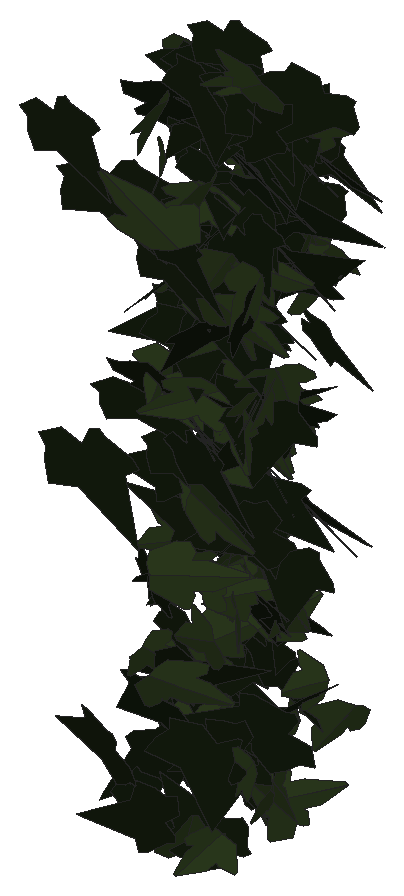
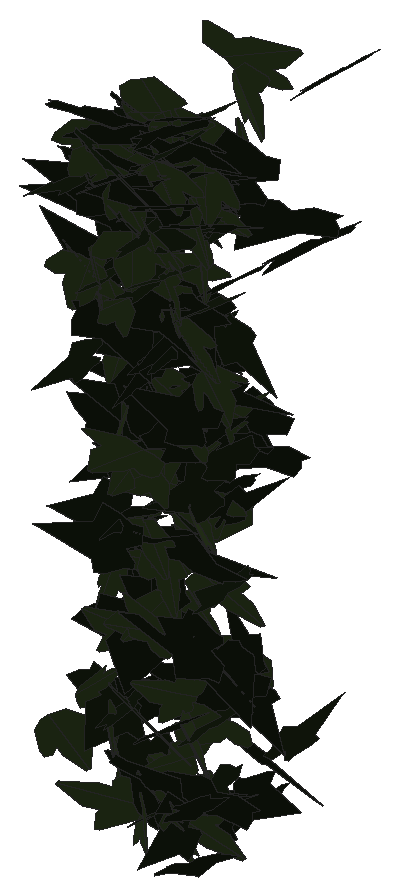
# SketchUp Ruby script. Lengths in millimetres.
U = 1.mm
M = Sketchup.active_model
def pt(a) = Geom::Point3d.new(a.map { |v| v * U })
def face(e, loops, mat)
  f = e.add_face(loops[0].map { |a| pt(a) })
  loops[1..].each { |l| e.add_face(l.map { |a| pt(a) }).erase! }
  f.material = f.back_material = mat if mat
  f
end
# faces: each face lists its corners as indices into pts; further lists are holes
def faces(e, pts, list, mat = nil) = list.each { |f| face(e, (f[0].is_a?(Array) ? f : [f]).map { |l| l.map { |i| pts[i] } }, mat) }
# xy, xz, yz: faces in a plane at the given z, y or x. An outline is a flat list of corners, or four numbers for a rectangle; further outlines are holes
def ring(l) = l.size == 4 ? [[l[0], l[1]], [l[2], l[1]], [l[2], l[3]], [l[0], l[3]]] : l.each_slice(2).to_a
def flat(e, list, mat, &to3) = list.each { |f| face(e, (f[0].is_a?(Array) ? f : [f]).map { |l| ring(l).map { |u, v| to3.(u, v) } }, mat) }
def xy(e, z, list, mat = nil) = flat(e, list, mat) { |x, y| [x, y, z] }
def xz(e, y, list, mat = nil) = flat(e, list, mat) { |x, z| [x, y, z] }
def yz(e, x, list, mat = nil) = flat(e, list, mat) { |y, z| [x, y, z] }
def lines(e, pts, list) = list.each { |a, b| e.add_line(pt(pts[a]), pt(pts[b])) }
# prism: a flat outline (further loops are holes) pulled along v
def prism(e, loops, v, mat = nil)
  f = face(e, loops, mat); d = Geom::Vector3d.new(v.map { |x| x * U })
  f.pushpull(f.normal.samedirection?(d) ? d.length : -d.length)
end
def box(e, o, s, mat = nil) = prism(e, [[o, [o[0] + s[0], o[1], o[2]], [o[0] + s[0], o[1] + s[1], o[2]], [o[0], o[1] + s[1], o[2]]]], [0, 0, s[2]], mat)
def at(x, y, z, deg = 0) = Geom::Transformation.translation(pt([x, y, z])) * Geom::Transformation.rotation(ORIGIN, Z_AXIS, deg.degrees)
def axes(o, x, y, z) = Geom::Transformation.new([*x, 0, *y, 0, *z, 0, *pt(o).to_a, 1])
def part(name) = M.definitions.add(name)
# library, detail: a bought-in or finely detailed component or shape, given as its bounding box
def library(name, o, s) = part(name).tap { |d| box(d.entities, o, s) }
def detail(e, o, s) = box(e.add_group.entities, o, s)
def put(e, d, t, mat = nil) = e.add_instance(d, t).tap { |i| i.material = mat if mat }
def group(e, t, mat = nil) = e.add_group.tap { |g| g.transformation = t; g.material = mat if mat }.entities
root = M.entities
M.materials.add("efeu1").color = [18, 25, 13]
M.materials.add("efeu2").color = [43, 57, 29]
c1 = part("ivyleaf_9")
p = [[39.1,54.8,31.7],[34.5,51.8,30.2],[-5.3,25.2,17.3],[-17.9,28.3,20.9],[-21.6,21.7,17],[-20.2,4.3,5.3],
  [-22.9,-0.3,2.5],[-17.1,-4,-0.6],[-2,-2.1,-1.2],[-0.7,-15.4,-10.1],[16.6,-22.3,-16.7],[21.1,-15.1,-12.5],
  [32.7,-10.7,-11],[46.1,-1.8,-6.6],[30.8,11.2,3.8]]
faces(c1.entities,p,[[0,1,2,3,4,5,6,7,8,9,10,11,12,13,14]],"efeu1")
c2 = part("ivyleaf_10")
p = [[0,12.8,-0.8],[-1.5,51.3,-10.9],[-4.9,51,-11.6],[-13.6,26.5,-7.3],[-13.2,15.9,-4.6],[-21.1,19.3,-7.2],
  [-29.5,16.3,-8.3],[-29.2,8.3,-6.2],[-19.7,-9.8,0.5],[-7.6,-13,4],[1,-12.2,5.8],[-0.4,51.1,-11.1],
  [-1.5,51.1,-10.9],[1,-12.4,5.9],[16.9,-12.4,3.5],[35.1,9.1,-5.1],[35,12.9,-6.1],[20.5,16.4,-4.9],
  [15.8,15,-3.8],[15.3,27.6,-7.1],[12.8,31.3,-7.8]]
faces(c2.entities,p,[[0,1,2,3,4,5,6,7,8,9,10],[11,12,0,13,14,15,16,17,18,19,20]],"efeu2")
put(root,c1,axes([3720.9,828.8,1939.2],[0.32232,0.88596,-0.48783],[-0.15644,-0.48093,-0.90196],[-1.9185,0.18806,-0.00841]))
put(root,c2,axes([3705.6,866.7,2568],[1.66073,-0.52387,-0.15282],[0.12616,0.38784,-0.951],[1.03089,0.79647,0.36257]))
put(root,c2,axes([3717.3,848.8,2294.4],[-0.3776,-0.95037,0.21572],[-0.04956,-0.21489,-0.97069],[1.85409,-0.19929,0.01799]))
put(root,c1,axes([3717,710.5,1766.5],[0.64465,-1.06589,-0.12588],[0.1178,-0.11238,1.11814],[-2.0393,-0.34343,0.0248]))
put(root,c1,axes([3691.6,852.7,2037.4],[0.40267,-0.965,0.20893],[0.08086,-0.20457,-0.98792],[1.87739,0.21579,-0.00226]))
put(root,c1,axes([3712.1,873.7,2507.2],[-1.16359,-0.7967,0.11583],[0.21549,-0.22909,-0.97808],[1.517,-0.57855,0.22778]))
put(root,c1,axes([3696.9,804.5,1925],[-0.07069,0.01892,0.92509],[0.31832,-0.91044,0.02533],[1.73198,0.1681,0.0331]))
put(root,c1,axes([3729.7,881.9,1758.7],[-0.10608,-0.69209,-0.58924],[-0.03591,-0.58934,0.69399],[-1.72954,0.05469,0.02173]))
put(root,c2,axes([3743.2,857.1,2500.2],[-0.75448,0.28971,0.97126],[-1.48217,0.58041,-0.49098],[-1.23457,-0.87386,-0.00411]))
put(root,c1,axes([3696.8,734.6,2469.4],[-0.49241,-0.85282,-0.81291],[0.58654,0.75431,-0.88944],[2.16425,-0.39846,0.0561]))
put(root,c1,axes([3734.4,795,2331.4],[-0.77181,0.79059,-0.42816],[0.34399,-0.38843,-0.88841],[-1.67621,-0.44374,0.01483]))
put(root,c1,axes([3698.9,775.5,2186.7],[-0.28847,-0.48267,-0.84014],[0.76914,0.74136,-0.49883],[1.67599,-0.4233,0.08432]))
put(root,c1,axes([3726,790.5,1736.2],[-0.05618,-0.06564,-1.18238],[0.72034,-1.12123,0.0528],[-2.13555,-0.37647,0.04891]))
put(root,c1,axes([3717,884.5,1697],[-0.59468,-0.89852,0.09086],[-0.05707,-0.08576,-0.9513],[1.71783,-0.3139,-0.00015]))
put(root,c1,axes([3741.7,843.7,1954.2],[-1.75891,0.45294,-0.32855],[0.56549,-0.14028,-1.0292],[-0.90239,-0.97076,-0.00457]))
put(root,c2,axes([3754,802.2,2004.5],[-1.07869,0.00415,0.74017],[-1.34345,-0.28349,-0.53894],[0.42381,-0.8881,0.17549]))
put(root,c2,axes([3755,847.3,1720.2],[-0.83308,-0.25611,0.80676],[-1.27743,-0.44833,-0.5065],[0.98148,-0.80091,0.02555]))
put(root,c1,axes([3755.7,825.3,2265.5],[-1.5034,-0.22021,0.56102],[-1.0224,-0.16203,-0.81999],[0.51999,-0.95524,0.00976]))
put(root,c2,axes([3736.4,837.2,2444.5],[0.49144,-0.48953,-0.86004],[-0.26953,0.86141,-0.53283],[1.86402,0.25362,0.1497]))
put(root,c1,axes([3705.3,855.4,1778],[-0.55905,-0.31991,-0.87643],[1.21772,0.59967,-0.43333],[1.29235,-0.70343,0.02918]))
put(root,c1,axes([3707.2,622.7,2600.8],[0.58457,-1.0927,-0.39439],[-0.12329,0.3912,-1.1343],[2.2075,0.31121,0.04109]))
put(root,c1,axes([3735.3,863.2,2557.2],[-1.33625,-0.7243,0.2139],[-0.10541,-0.24189,-1.00087],[1.43348,-0.69296,0.12579]))
put(root,c1,axes([3744.6,789.9,2090.9],[-0.34654,-0.06798,1.00578],[-1.2974,-0.74464,-0.17374],[1.41339,-0.70019,0.08711]))
put(root,c2,axes([3726,787.4,2222.1],[-0.38352,-0.6161,0.84039],[0.68759,-0.84418,-0.53224],[1.86019,0.18501,0.37]))
put(root,c1,axes([3719.6,848.7,1852.6],[-0.12427,-0.97947,0.57005],[-0.08648,-0.56827,-0.98162],[2.15511,-0.07928,-0.00652]))
put(root,c1,axes([3734.2,851.3,2379.2],[-0.65697,-0.75817,0.56128],[-0.13996,-0.57423,-0.82089],[1.78987,-0.32319,0.14183]))
put(root,c1,axes([3698.8,878.7,1973.8],[0.87885,0.1007,-0.92747],[1.73885,0.16047,0.47232],[0.35907,-1.02357,-0.0172]))
put(root,c1,axes([3728.7,733.7,1713],[0.58804,-0.65489,-0.66012],[-0.47987,0.61055,-0.72372],[1.70341,0.39808,0.024]))
put(root,c1,axes([3757.1,800.8,1705.8],[0.38753,-0.3916,0.81944],[-0.53444,0.77149,0.43846],[-1.64379,-0.34315,0.05063]))
put(root,c1,axes([3719.3,821.8,1765],[1.05612,-0.81786,-0.1043],[-0.11772,0.08407,-0.98834],[1.56473,0.55834,-0.00396]))
put(root,c2,axes([3761.2,847.5,2346.8],[1.25686,-0.42115,-0.66754],[-0.95638,0.44685,-0.77904],[1.1584,0.82587,0.0811]))
put(root,c1,axes([3716.4,807.3,2173.9],[0.50475,-0.70377,0.63807],[0.54289,-0.57289,-0.75045],[1.72453,0.38634,0.04949]))
put(root,c1,axes([3709.8,879.7,2255.2],[0.80111,-0.46544,0.73818],[0.97657,-0.53091,-0.62735],[1.34341,0.66349,0.01585]))
put(root,c2,axes([3738.8,745.7,1885.5],[-0.39761,-0.62362,-0.72993],[0.64035,0.65207,-0.65341],[1.71128,-0.3889,0.0749]))
put(root,c1,axes([3770.3,728.3,1838.8],[0.55397,0.14839,-0.92399],[-1.74786,-0.14072,-0.3119],[-0.34237,0.95848,0.09726]))
put(root,c1,axes([3702.2,797.4,2536],[0.99853,-0.06465,0.98926],[1.87393,-0.0964,-0.5285],[0.21979,1.11562,0.01166]))
put(root,c1,axes([3761.1,845.9,2051],[-1.99883,0.14244,0.21134],[0.3962,-0.03756,1.05982],[0.27984,1.07064,0.00906]))
put(root,c1,axes([3707.2,769.6,2200.7],[0.73076,-0.25382,0.87054],[1.57825,-0.28418,-0.44861],[0.69821,0.90802,0.10294]))
put(root,c2,axes([3746.1,848.9,1834],[0.99743,-1.03025,0.2683],[0.21992,-0.24223,-1.15587],[2.01419,0.53663,-0.00665]))
put(root,c2,axes([3727.9,821.4,1845.8],[1.63827,0.16369,0.43784],[0.82382,0.06714,-0.87612],[-0.33576,0.96341,-0.01333]))
put(root,c2,axes([3738.7,844.2,2541],[-1.29681,0.48042,-0.54987],[0.63075,-0.46669,-0.81842],[-1.23828,-0.74084,0.15898]))
put(root,c2,axes([3751.6,828.4,2101.8],[0.5869,-0.88463,0.29249],[0.16232,-0.27999,-0.93678],[1.76583,0.31976,-0.0111]))
put(root,c1,axes([3761.1,821.3,2545.1],[-1.66196,0.16856,-0.48498],[0.86781,-0.18524,-0.88541],[-0.44918,-0.98155,0.08382]))
put(root,c1,axes([3789.9,798,2026.7],[-0.54505,0.3559,0.81761],[-1.52715,0.27173,-0.39934],[-0.74027,-0.8226,0.22183]))
put(root,c2,axes([3743.1,780.9,2197.9],[0.59955,0.84677,0.37219],[0.28112,0.34208,-0.9033],[-1.73779,0.34748,-0.01772]))
put(root,c1,axes([3741.8,862,1722.5],[1.50212,-0.39965,-0.35194],[-0.58737,0.16952,-0.88461],[0.82594,0.84738,0.01098]))
put(root,c1,axes([3760.2,874.5,2514.7],[-1.21239,-0.7684,0.18306],[0.05837,-0.25906,-0.98067],[1.50222,-0.61008,0.18585]))
put(root,c1,axes([3774.5,845.5,2371.9],[0.76965,0.54385,-0.7747],[-0.8032,-0.65047,-0.67694],[-1.61248,0.58359,-0.03258]))
put(root,c1,axes([3780.2,844.6,2188.4],[-0.08212,-0.05191,1.03692],[-1.71879,-0.51007,-0.06312],[0.97471,-0.90382,-0.02394]))
put(root,c1,axes([3744,786.5,2128.4],[0.23205,-0.85642,-0.46133],[-0.05055,0.46184,-0.86438],[1.85069,0.11999,0.03424]))
put(root,c1,axes([3779.1,865.2,2528.6],[-1.48089,-0.5283,0.39865],[-0.61494,-0.23376,-0.94044],[1.09929,-0.84245,0.01096]))
put(root,c1,axes([3753.6,859.2,2559.2],[-1.03992,-0.77859,-0.31056],[0.46609,0.20626,-0.948],[1.52575,-0.59369,0.07792]))
put(root,c1,axes([3732.2,862.7,2485.4],[0.79504,-0.85171,0.28529],[0.59688,-0.15653,-0.92652],[1.6019,0.48103,0.20364]))
put(root,c2,axes([3766.4,848.5,1711.1],[1.11606,-0.77525,-0.09309],[-0.10724,0.07411,-0.97206],[1.48218,0.58911,-0.00023]))
put(root,c1,axes([3768.1,851.9,2581.3],[-1.69898,-0.44177,-0.30747],[0.51803,0.14318,-0.996],[0.88372,-0.93324,-0.00727]))
put(root,c1,axes([3737.5,822.3,2137],[1.50595,-0.62138,0.00652],[0.0067,-0.00608,-1.00609],[1.18266,0.79128,-0.0026]))
put(root,c2,axes([3772.6,792.1,2311.4],[0.2658,-0.75749,-0.81498],[-0.12046,0.81464,-0.76802],[2.11417,0.14165,0.05871]))
put(root,c1,axes([3750.8,822.8,2327],[0.1518,-0.092,-1.02629],[-0.12327,1.02688,-0.09708],[1.95719,0.07181,0.07348]))
put(root,c1,axes([3747.4,870.6,2592.9],[0.29906,-1.01272,0.00254],[0.00043,-0.00253,-1.02483],[1.92741,0.15714,-0.00016]))
put(root,c1,axes([3747.1,769.3,2381],[0.34188,-1.05627,-0.2565],[-0.04309,0.25628,-1.07125],[2.06827,0.17994,0.02008]))
put(root,c2,axes([3742.6,852.7,2223.9],[1.06818,-0.3845,0.69192],[1.25117,-0.24606,-0.66998],[0.83918,0.85628,0.11817]))
put(root,c2,axes([3767.5,874.7,2558.9],[1.86393,-0.22116,-0.12808],[-0.2098,0.0921,-1.00192],[0.43883,0.9834,0.06503]))
put(root,c1,axes([3763,798.5,2274.3],[-0.67454,-0.99544,-0.08466],[0.05914,0.0788,-1.05665],[1.90044,-0.35577,0.00284]))
put(root,c1,axes([3770.3,868.1,1840.1],[-0.56943,-0.83094,0.40734],[-0.21879,-0.39141,-0.88288],[1.74759,-0.31975,0.02219]))
put(root,c1,axes([3754.9,861,2613],[0.14073,-0.93447,-0.38706],[0.15532,0.39234,-0.93162],[1.91872,0.03678,0.1038]))
put(root,c2,axes([3778.1,713.5,2592.8],[0.32725,-1.20083,0.0992],[0.05121,-0.09636,-1.21301],[2.29263,0.17356,0.01293]))
put(root,c2,axes([3805.8,818.6,2247.4],[0.31853,-0.23559,-1.0808],[-1.32813,0.82565,-0.28804],[1.63349,0.71725,-0.02344]))
put(root,c1,axes([3791.3,838.1,2349.2],[-1.38537,-0.62121,0.29921],[-0.40277,-0.2128,-0.95667],[1.24894,-0.7577,0.02338]))
put(root,c2,axes([3785.3,710.2,2528.9],[0.40211,-0.76936,-0.68755],[-0.11812,0.69107,-0.79237],[1.96019,0.19947,0.0933]))
put(root,c2,axes([3778.5,830.6,2364.1],[0.2883,-0.92723,0.34655],[0.25428,-0.32822,-0.9366],[1.86668,0.18791,0.07406]))
put(root,c1,axes([3755.9,878.2,2429.4],[0.34,-0.96038,-0.15125],[0.33076,0.18285,-0.95577],[1.82053,0.14614,0.20189]))
put(root,c2,axes([3801.2,765.8,2216.5],[0.84925,0.3457,-0.90075],[-1.44808,-0.48413,-0.56273],[-1.12906,0.88095,0.04422]))
put(root,c1,axes([3744.3,762.6,1847.1],[0.57014,0.02723,1.04417],[1.94459,0.21799,-0.29882],[-0.41291,1.0642,0.03449]))
put(root,c2,axes([3779.3,800.2,2106.5],[2.01494,0.30675,-0.19017],[-0.3469,-0.05426,-1.10226],[-0.59287,1.07429,-0.00137]))
put(root,c1,axes([3815.2,672.8,1725.8],[-1.43628,0.54052,0.38731],[-0.59147,0.23124,-0.92825],[-1.11884,-0.81613,-0.00649]))
put(root,c2,axes([3764.5,833,1872],[0.39671,0.31534,-0.9882],[1.16514,0.77628,0.37685],[1.59368,-0.64604,-0.02953]))
put(root,c2,axes([3808.7,829.1,2395.4],[-1.16733,0.39923,0.74009],[-1.28419,0.31301,-0.72805],[-0.95508,-0.90883,0.07436]))
put(root,c2,axes([3802.9,772.2,2461.4],[1.14519,0.38608,-0.75551],[-1.28766,-0.34054,-0.71287],[-0.97435,0.90382,0.05413]))
put(root,c1,axes([3811.4,852.6,1756.8],[-2.03032,0.20701,-0.21356],[-0.40076,0.0359,1.08668],[0.39976,1.08736,0.00478]))
put(root,c2,axes([3805.4,855,2077.2],[-1.34339,0.30113,0.51014],[-0.97616,0.08637,-0.76067],[-0.56409,-0.86661,0.10145]))
put(root,c2,axes([3779.8,869.9,2465.7],[1.36379,-0.64273,0.24249],[0.30885,-0.18211,-0.96223],[1.2704,0.73425,-0.02639]))
put(root,c2,axes([3797.1,819.9,2582.3],[-0.64234,-0.95975,0.26741],[-0.03501,-0.27629,-1.01482],[1.89584,-0.33028,0.07186]))
put(root,c1,axes([3762.9,850.1,2520.3],[1.13471,0.23261,0.76126],[1.29707,0.34226,-0.63834],[-0.78275,0.90435,0.04578]))
put(root,c2,axes([3783.8,768.4,1781.8],[0.56795,0.56117,-0.90359],[0.69564,0.82723,0.63446],[1.9011,-0.47034,0.03779]))
put(root,c2,axes([3782.6,811.7,1773.4],[-0.08372,-0.05123,-1.07154],[0.88895,0.96454,-0.06528],[1.83801,-0.46883,-0.01723]))
put(root,c2,axes([3799.8,840.5,1738.4],[1.23801,-0.76511,-0.13929],[-0.16867,0.10748,-1.00426],[1.47045,0.6565,0.00208]))
put(root,c1,axes([3782.8,803,2582.6],[-0.3214,-1.1325,0.35966],[0.03082,-0.36543,-1.14308],[2.26125,-0.15598,0.0667]))
put(root,c1,axes([3777.5,827.7,1737.1],[0.79178,-0.94136,-0.35014],[-0.23327,0.32858,-1.029],[1.89723,0.43326,0.01961]))
put(root,c1,axes([3776.4,872.3,2418.4],[1.02446,-0.80602,-0.202],[-0.17211,0.18243,-0.9689],[1.57207,0.54523,0.02556]))
put(root,c1,axes([3823.9,872.1,1864.7],[-1.53459,0.58689,-0.0241],[0.02255,-0.02466,-0.99721],[-1.11769,-0.80631,0.01296]))
put(root,c2,axes([3819.6,806.5,2014.5],[-1.4459,0.51567,0.63935],[-1.06814,0.31001,-0.91693],[-1.14144,-0.94331,0.04816]))
put(root,c2,axes([3827.8,741.9,1927.9],[-0.76744,0.32257,0.85143],[-1.53309,0.30764,-0.49805],[-0.80768,-0.89044,0.13637]))
put(root,c2,axes([3812.1,788.7,2381.9],[-1.19808,-0.76609,0.26512],[-0.29363,-0.21632,-0.9914],[1.51467,-0.6479,0.01752]))
put(root,c2,axes([3779,724.5,1870.6],[-0.91565,-0.36705,-0.98062],[1.45972,0.61111,-0.60504],[1.35659,-0.90532,-0.01084]))
put(root,c2,axes([3799.4,811.1,1744],[0.28373,-0.77037,0.57617],[-0.16963,0.56948,0.78449],[-1.82301,-0.17289,0.01668]))
put(root,c2,axes([3800.9,737.9,1661],[-0.76563,-0.88847,-0.15277],[-0.07575,-0.14962,0.97498],[-1.71408,0.40347,0.02515]))
put(root,c1,axes([3796.4,831,2294.2],[0.55413,-0.37408,-0.94032],[-0.7601,0.85657,-0.46442],[1.7697,0.48504,0.09496]))
put(root,c2,axes([3811.4,871.8,2447.4],[-1.57771,-0.58294,-0.0186],[0.02122,0.01647,-1.0134],[1.10982,-0.82902,-0.00706]))
put(root,c1,axes([3777.9,729.3,2430.5],[0.96344,-1.09194,-0.01958],[-0.0105,0.01902,-1.20357],[2.07849,0.50624,0.003]))
put(root,c1,axes([3790.7,801.2,2476.5],[-0.21612,-0.95344,0.41896],[0.10545,-0.42638,-0.9553],[1.97924,-0.08139,0.09664]))
put(root,c2,axes([3821.1,790.7,2304.2],[-1.01357,-0.50496,0.77421],[-0.43399,-0.79413,-0.67481],[1.70481,-0.50238,0.28851]))
put(root,c1,axes([3788,818.7,2440.3],[0.27991,-0.93718,-0.37445],[0.0794,0.38373,-0.94401],[1.9191,0.12081,0.09367]))
put(root,c1,axes([3784.6,875.7,2470.9],[0.74991,-0.92841,-0.05768],[0.02602,0.06842,-1.0078],[1.77016,0.39231,0.03925]))
put(root,c1,axes([3808,820.5,2565.7],[-1.39613,-0.65535,-0.20186],[0.40242,0.06502,-0.9795],[1.24149,-0.75806,0.09049]))
put(root,c1,axes([3822.4,749.6,2317.2],[-0.25896,0.85879,-0.68034],[0.23974,-0.66876,-0.86936],[-2.07135,-0.18477,-0.01556]))
put(root,c1,axes([3832.2,753.6,1663.7],[-1.50012,-0.6818,0.16491],[0.24419,0.10375,1.04216],[-1.31251,0.79857,0.00541]))
put(root,c2,axes([3840.9,807.6,2602.8],[-1.44395,0.15917,0.7499],[-1.42148,0.08426,-0.77354],[-0.32876,-1.06342,0.05095]))
put(root,c2,axes([3820.6,877.3,2514.9],[-0.47178,-0.91344,0.329],[0.04035,-0.34457,-0.94068],[1.84734,-0.22575,0.10457]))
put(root,c2,axes([3835.6,823.5,1693.5],[-0.20546,0.14861,1.08255],[-1.28625,0.84572,-0.1835],[-1.63416,-0.68435,0.00832]))
put(root,c2,axes([3837.2,812.2,2346.1],[-0.19032,0.19695,-1.11766],[-0.76741,1.04262,0.21981],[2.01897,0.41486,-0.02181]))
put(root,c1,axes([3802.2,832.8,1698],[-0.77935,0.55901,0.83051],[0.82147,-0.71104,0.69141],[1.71915,0.59318,0.04612]))
put(root,c2,axes([3811.3,819.6,1963.5],[-0.52396,-0.6108,-0.79172],[0.77664,0.68106,-0.66732],[1.73742,-0.48864,0.05954]))
put(root,c2,axes([3784.6,863.7,1959.4],[0.93364,-0.06759,0.9252],[1.7521,-0.09337,-0.49495],[0.21734,1.04304,0.01565]))
put(root,c1,axes([3790.6,840.8,2317.8],[1.54641,-0.63803,0.13642],[0.20405,-0.08435,-1.0331],[1.22487,0.81957,-0.00013]))
put(root,c2,axes([3807.2,850.9,2149.4],[-1.45176,0.29015,-0.52841],[0.81979,-0.33387,-0.80514],[-0.80265,-0.8658,0.1334]))
put(root,c2,axes([3819.7,761.6,1998.6],[0.25059,-0.22042,0.96227],[-0.20031,0.96213,0.23479],[-1.86812,-0.13273,0.1039]))
put(root,c1,axes([3828,824.5,2574.1],[-1.20163,-0.80957,0.35535],[-0.2734,-0.33692,-1.02282],[1.6603,-0.6414,0.08876]))
put(root,c1,axes([3817,786.6,2171.3],[1.38708,-0.37273,-0.58808],[-0.9833,0.28116,-0.8185],[0.88826,0.89328,0.01224]))
put(root,c2,axes([3806.5,801.5,2569.4],[0.77715,0.68659,0.64921],[0.6161,0.56279,-0.79881],[-1.68955,0.52104,0.00733]))
put(root,c1,axes([3825,839.7,2059.8],[-0.89137,-0.89364,0.00731],[-0.00232,-0.00761,-1.00893],[1.70083,-0.46835,0.00246]))
put(root,c1,axes([3816.6,864.1,2528.3],[-0.47411,-0.94187,-0.24289],[0.1839,0.22553,-0.97363],[1.84205,-0.26493,0.03469]))
put(root,c1,axes([3846.7,791,1760.8],[-0.102,1.11353,-0.19815],[-0.02408,-0.19895,-1.11461],[-2.15243,-0.05054,0.02186]))
put(root,c2,axes([3818,787.2,2324.9],[-1.26055,0.54916,-0.48793],[0.57159,-0.39713,-0.85465],[-1.27592,-0.72045,0.09919]))
put(root,c1,axes([3842.7,861.3,2345.3],[0.54532,0.70685,-0.6284],[-0.37542,-0.5975,-0.76204],[-1.76045,0.34637,-0.03215]))
put(root,c2,axes([3839.3,737.2,1679.9],[0.6313,0.53207,-0.78016],[-0.77,-0.66708,-0.62697],[-1.62393,0.52314,-0.006]))
put(root,c2,axes([3824.8,835.9,2158.4],[-1.02816,-0.6968,-0.55772],[0.70542,0.41791,-0.88114],[1.54523,-0.65442,0.03116]))
put(root,c2,axes([3838.7,718.8,2510.9],[0.14314,-1.21297,0.05991],[0.01021,-0.05969,-1.2153],[2.31132,0.07538,0.00166]))
put(root,c1,axes([3847.8,813.8,2160.4],[-0.18885,0.41129,-0.95314],[0.13667,-0.95247,-0.41847],[-1.97095,-0.10546,0.06231]))
put(root,c1,axes([3846.2,754.1,2457.5],[-0.86205,0.68125,-0.58517],[0.55066,-0.50975,-0.81739],[-1.61807,-0.53642,0.03359]))
put(root,c2,axes([3839.3,826.7,2337.7],[-0.31427,-1.04166,-0.11128],[0.03138,0.11006,-1.05467],[1.99352,-0.16595,-0.00094]))
put(root,c1,axes([3833.7,826.2,1938.1],[1.63045,0.54437,-0.40831],[-0.67319,-0.20457,-1.01489],[-1.10638,0.9267,0.01581]))
put(root,c1,axes([3873.4,795.4,2562.9],[-1.49713,0.6294,0.42305],[-0.67053,0.23647,-1.00692],[-1.27812,-0.86131,0.03271]))
put(root,c1,axes([3815.4,861.9,1858],[0.92421,-0.94616,-0.30487],[-0.27076,0.26967,-1.0635],[1.87244,0.50601,-0.0033]))
put(root,c2,axes([3812.3,867.1,2179.8],[1.35971,0.30335,0.61866],[1.0288,0.30587,-0.77422],[-0.81318,0.8942,0.05495]))
put(root,c1,axes([3814.3,794.1,1947.6],[1.44149,0.30109,0.46491],[0.77156,0.23533,-0.81285],[-0.71832,0.85699,0.05987]))
put(root,c1,axes([3826.2,789.2,2314.1],[-0.98014,-0.678,-0.63615],[0.68794,0.52399,-0.85109],[1.63022,-0.62876,-0.02332]))
put(root,c2,axes([3841.1,731.7,2003.1],[0.08368,0.12404,0.98906],[-0.40051,0.96886,-0.11215],[-1.85436,-0.20366,0.06885]))
put(root,c2,axes([3816.4,816,2170.1],[-1.28433,0.42661,-0.8087],[1.21513,-0.49959,-0.79633],[-1.2456,-0.92725,0.05699]))
put(root,c1,axes([3829.6,810.5,2340.2],[-0.18509,-0.35412,0.97283],[-0.14585,-0.97197,-0.36147],[1.96493,-0.1055,0.0648]))
put(root,c2,axes([3809.7,691.9,2029.4],[0.21971,-0.1362,-1.174],[1.78929,0.7254,0.00829],[1.36308,-0.93027,0.17835]))
put(root,c1,axes([3830.9,876.4,2525.3],[-0.38485,-0.98144,0.1434],[0.02166,-0.14864,-1.00123],[1.88759,-0.19839,0.04073]))
put(root,c1,axes([3861.1,754.9,2076.1],[-1.01142,0.81805,-0.2085],[0.23426,-0.16865,-0.97545],[-1.58952,-0.54539,-0.0111]))
put(root,c1,axes([3810.8,759.4,2159.4],[1.07379,-0.45128,-0.97687],[1.68217,-0.43479,0.71134],[-1.16814,-1.04094,0.12639]))
put(root,c2,axes([3830.8,874.2,2370.7],[-1.25069,0.56335,-0.47401],[0.71964,-0.28693,-0.86521],[-1.20229,-0.75776,-0.02478]))
put(root,c1,axes([3871.5,870.1,2556.8],[-1.33224,0.74436,0.00306],[-0.02602,-0.00866,-1.02167],[-1.41644,-0.69995,0.0159]))
put(root,c1,axes([3824.2,790.7,2339.2],[-0.84544,0.38361,0.92445],[1.23606,-0.65908,0.58558],[1.44938,0.78584,0.03985]))
put(root,c2,axes([3848.7,792.3,2218.8],[0.08174,-0.99561,0.12288],[0.09989,-0.1206,-0.99543],[1.90661,0.049,0.04689]))
put(root,c1,axes([3830.5,801.5,2459.7],[0.09674,-0.96506,-0.23992],[0.01678,0.24066,-0.96617],[1.89253,0.0472,0.02083]))
put(root,c2,axes([3855.3,871.1,2544.5],[-1.28785,-0.7453,0.17455],[-0.07234,-0.19997,-1.0012],[1.45504,-0.66961,0.10472]))
put(root,c2,axes([3829.3,788.7,1966.2],[0.5908,-0.7438,0.84573],[1.08021,-0.65442,-0.78387],[1.85145,0.61916,0.18747]))
put(root,c1,axes([3866.5,866.4,2502],[-1.46234,0.60828,-0.2117],[0.34293,-0.11336,-0.97973],[-1.17683,-0.78888,-0.02244]))
put(root,c1,axes([3821.1,804.7,2190.9],[0.71919,0.94149,-0.40292],[0.15749,0.4,1.01228],[1.94267,-0.38098,0.0671]))
put(root,c1,axes([3842.9,789.9,1968],[1.52465,-0.12733,-0.47848],[-0.90651,0.0504,-0.81087],[0.25738,0.93175,-0.02153]))
put(root,c1,axes([3869.8,871.2,2541.3],[-1.86183,-0.27368,0.10726],[-0.19697,-0.0282,-1.01583],[0.52363,-0.98372,-0.00072]))
put(root,c2,axes([3854.5,792.3,2223.7],[0.5282,-0.94116,-0.40182],[-0.06861,0.40708,-0.97839],[1.94642,0.26975,0.07455]))
put(root,c1,axes([3836.4,817.1,2079.9],[-0.3262,-1.08547,-0.1402],[0.06933,0.13617,-1.09882],[2.08188,-0.17461,0.01463]))
put(root,c1,axes([3843.1,834.4,2185.6],[1.81699,-0.03705,0.46223],[-0.87931,0.01426,0.95541],[-0.0753,-1.06061,-0.0033]))
put(root,c1,axes([3879,732.1,1813.2],[-1.66296,0.49225,-0.00129],[0.00326,0.00042,-1.00289],[-0.93685,-0.87377,-0.0012]))
put(root,c1,axes([3825.2,803.9,1957.6],[-0.00142,-0.33269,1.07237],[0.8311,-0.98803,-0.30622],[1.96866,0.41687,0.13005]))
put(root,c1,axes([3838.1,816.9,2568.7],[0.0375,-0.96646,-0.33025],[0.02002,0.33048,-0.96652],[1.94369,0.01524,0.01633]))
put(root,c2,axes([3867.2,841.1,1807.8],[0.06649,-0.21739,-1.01749],[-0.4433,0.9906,-0.21964],[1.92994,0.23502,-0.01539]))
put(root,c1,axes([3892.1,790.3,1813.6],[-0.53608,-0.37531,-1.00841],[-1.22049,-0.77847,0.46886],[-1.64437,0.70015,-0.01924]))
put(root,c2,axes([3856.7,835.8,2199.4],[-0.91685,0.80136,0.12608],[-0.15526,0.09804,-0.93482],[-1.53608,-0.48822,0.01923]))
put(root,c1,axes([3839.2,836.1,2495.9],[-0.01615,-0.90775,0.46827],[0.16337,-0.46727,-0.90424],[1.93708,0.03184,0.08017]))
put(root,c2,axes([3836.4,776.4,2190.9],[1.2014,-0.36967,0.66999],[1.06618,-0.36841,-0.73108],[0.99208,0.84359,-0.02567]))
put(root,c1,axes([3837.9,872.9,2401],[0.34113,-0.96788,0.04189],[0.11413,-0.03144,-0.9829],[1.84026,0.18137,0.05319]))
put(root,c1,axes([3854.4,721.1,1813.1],[-1.11809,-1.0267,-0.23131],[0.23102,0.19704,-1.18287],[1.98962,-0.59984,0.00736]))
put(root,c1,axes([3822.9,874.6,2058.3],[1.23953,-0.48232,0.57917],[0.93718,-0.30719,-0.80957],[1.08597,0.81562,0.03758]))
put(root,c2,axes([3889.3,584.8,2533.4],[1.62958,0.21164,0.86664],[-1.6175,-0.1717,0.8816],[0.5162,-1.20612,0.02657]))
put(root,c2,axes([3841.6,756.6,1984.9],[0.15875,0.08855,-1.05482],[1.32125,0.79418,0.12157],[1.52082,-0.6992,0.00449]))
put(root,c1,axes([3851.6,852.7,2570.6],[-0.58373,-0.89186,-0.40394],[0.27114,0.37813,-0.94307],[1.84354,-0.33801,0.0108]))
put(root,c2,axes([3844.1,825,1923],[0.75098,0.42653,-0.89712],[1.17422,0.65131,0.58103],[1.48169,-0.73234,-0.00577]))
put(root,c1,axes([3841.7,503.8,2281],[0.3803,-1.30026,-0.40579],[-0.03787,0.4073,-1.3149],[2.59209,0.19672,0.04032]))
put(root,c2,axes([3859,785.3,2042.2],[0.16032,0.91846,0.37096],[0.07549,0.36887,-0.9223],[-1.8837,0.09296,-0.00539]))
put(root,c1,axes([3846.9,779.1,2439.8],[-0.83517,-0.31892,-0.83636],[1.6767,0.01089,-0.46639],[0.30136,-0.94443,0.27705]))
put(root,c2,axes([3868.3,865.5,2404.2],[0.57901,-0.93063,-0.1595],[0.11259,0.18603,-0.97261],[1.79347,0.28877,0.11255]))
put(root,c1,axes([3834.7,804.3,2495.7],[0.90065,-0.6754,0.56397],[0.6342,-0.4551,-0.82464],[1.54991,0.5787,0.0097]))
put(root,c1,axes([3854.4,832.4,2536.3],[-0.17672,-1.03662,-0.03036],[0.00707,0.03014,-1.04077],[1.97373,-0.09292,0.00101]))
put(root,c1,axes([3839.4,820.5,2548],[1.57177,-0.62141,0.09302],[0.14068,-0.05648,-1.03353],[1.18754,0.82916,-0.00069]))
put(root,c1,axes([3868.6,784.8,2219.5],[-1.80163,-0.4547,-0.58605],[0.99501,0.26504,-1.05012],[1.00145,-1.08135,-0.01096]))
put(root,c1,axes([3903.1,751.9,2087.2],[-1.78076,-0.01956,0.33119],[-0.63046,0.00041,-0.93585],[0.03483,-0.99255,-0.00692]))
put(root,c1,axes([3875.2,819.1,1825],[0.6211,0.88829,0.60233],[0.39394,0.56565,-0.94634],[-2.00425,0.38645,0.00065]))
put(root,c2,axes([3850.7,745.3,2354.2],[-1.4491,0.07192,-0.74112],[1.39453,-0.11617,-0.76406],[-0.25206,-1.05617,0.03357]))
put(root,c1,axes([3828.1,813.8,2454.8],[0.9146,0.17396,-1.14382],[1.55957,0.82318,0.46947],[1.55444,-0.92824,0.20198]))
put(root,c1,axes([3892.3,846.3,2482],[-1.81478,-0.27346,-0.08998],[0.18535,-0.01344,-0.99119],[0.5156,-0.95768,0.03961]))
put(root,c1,axes([3859.6,816.2,2408.9],[1.68102,-0.52878,-0.31119],[-0.51132,0.15706,-1.02944],[1.04982,0.92321,-0.00311]))
put(root,c2,axes([3883,868.1,2390],[-1.74066,0.32449,0.01296],[-0.02135,0.00714,-0.97045],[-0.6177,-0.91466,-0.00298]))
put(root,c2,axes([3842.2,793.6,2384.6],[0.35515,-0.23896,-1.05542],[1.78158,-0.50166,0.27909],[-1.03323,-0.94714,0.11845]))
put(root,c2,axes([3851.7,826.3,1701.7],[0.48892,0.25622,-1.09402],[1.62717,0.68361,0.36087],[1.38758,-0.89193,-0.0377]))
put(root,c2,axes([3910.4,765.2,1732.4],[0.16108,-0.13184,-1.20356],[-1.31228,0.98649,-0.15655],[1.89414,0.69466,-0.00611]))
put(root,c1,axes([3864.7,810.2,2112],[-0.14125,-0.27151,1.00837],[0.15785,-1.00925,-0.26565],[1.9812,0.06105,0.09306]))
put(root,c1,axes([3852.4,851.6,2080.6],[1.16184,-0.68748,0.3372],[0.40544,-0.26174,-0.9193],[1.3998,0.64643,-0.01361]))
put(root,c1,axes([3844.4,869.4,2500.8],[1.05264,-0.49712,0.70228],[1.04443,-0.4392,-0.74309],[1.26125,0.77859,0.02922]))
put(root,c1,axes([3892,858.2,2587.1],[-1.68548,-0.51614,-0.03288],[0.24957,-0.16102,-1.00431],[0.95214,-0.87146,0.20504]))
put(root,c2,axes([3885.3,856.8,1845.9],[-0.35259,0.1902,0.96966],[0.2794,-0.97031,0.21838],[1.85975,0.18183,0.15103]))
put(root,c2,axes([3886.8,776.9,1743.1],[-0.12308,-0.7813,-0.75993],[0.26485,0.74912,-0.78203],[2.05736,-0.14318,0.05521]))
put(root,c2,axes([3847.1,702,2123.4],[0.27271,-0.13167,1.12732],[2.0652,-0.31721,-0.17498],[0.63325,1.09122,0.08517]))
put(root,c2,axes([3885.3,844.9,2550.4],[-1.40212,-0.62403,-0.29686],[0.43908,0.18693,-0.96547],[1.23974,-0.77197,0.00619]))
put(root,c2,axes([3886.1,789.9,2263.3],[-1.15388,-0.74749,-0.29267],[0.39696,0.20748,-0.96199],[1.4753,-0.64046,0.02994]))
put(root,c2,axes([3885.1,826.8,2337],[0.3756,-0.83656,0.62727],[-0.28676,0.60893,0.85951],[-1.96924,-0.24823,-0.00552]))
put(root,c2,axes([3886,775.6,2243.7],[-0.2299,0.38531,-0.91012],[-0.17123,-0.91737,-0.37644],[-1.87317,0.03657,0.14611]))
put(root,c1,axes([3866.1,660.5,2219.4],[1.10473,-1.04021,-0.20961],[-0.1619,0.19253,-1.19105],[2.01302,0.58634,0.01924]))
put(root,c1,axes([3904.1,707.7,2383.7],[-0.0152,-0.03304,-1.24456],[-1.5825,0.92646,-0.01926],[1.76355,0.83106,-0.02801]))
put(root,c1,axes([3872.9,869.3,2282.2],[1.27573,-0.622,-0.34601],[-0.36471,0.30004,-0.91059],[1.3046,0.69211,0.08379]))
put(root,c2,axes([3898.9,713.7,1806],[1.14071,-0.76134,-0.25243],[-0.2944,0.19949,-0.96896],[1.4979,0.619,0.00179]))
put(root,c1,axes([3870.2,771.6,2117.7],[0.04907,-0.44563,-0.93884],[0.45807,0.91615,-0.42826],[1.92409,-0.20675,0.1259]))
put(root,c2,axes([3906.5,883.3,1803.3],[-0.70979,-0.87684,0.45217],[-0.21354,-0.44256,-0.95076],[1.86545,-0.38429,0.06321]))
put(root,c2,axes([3871.1,862.1,2373.5],[0.06155,-0.35529,-0.92496],[1.0717,-0.75489,0.30965],[-1.55166,-0.53548,0.17718]))
put(root,c1,axes([3888.9,810,2030],[-0.56137,-1.09975,0.1703],[-0.07566,-0.16566,-1.13861],[2.11665,-0.2976,0.00447]))
put(root,c1,axes([3866,827.1,2367.5],[-0.36181,-0.12223,1.03276],[1.83008,-0.42052,0.12724],[0.75384,0.96223,0.1868]))
put(root,c1,axes([3873.5,869.4,2517.1],[1.04627,-0.81143,-0.30196],[-0.03963,0.3452,-0.96552],[1.64731,0.52368,0.16856]))
put(root,c2,axes([3895.7,798.1,1967.6],[-0.12498,-0.82595,-0.60665],[0.4042,0.58373,-0.81773],[1.90806,-0.17776,0.13349]))
put(root,c2,axes([3898.8,726,2407.7],[1.4144,-1.01173,0.08716],[0.09727,-0.07061,-1.25534],[1.9302,0.74492,-0.00061]))
